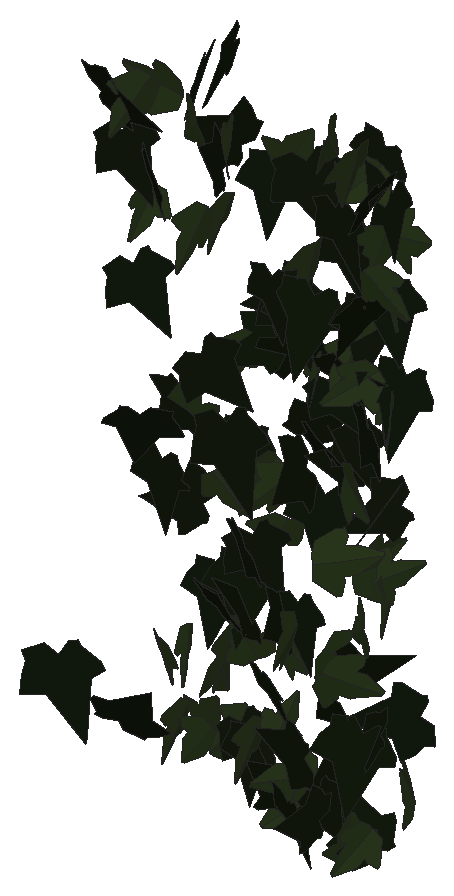
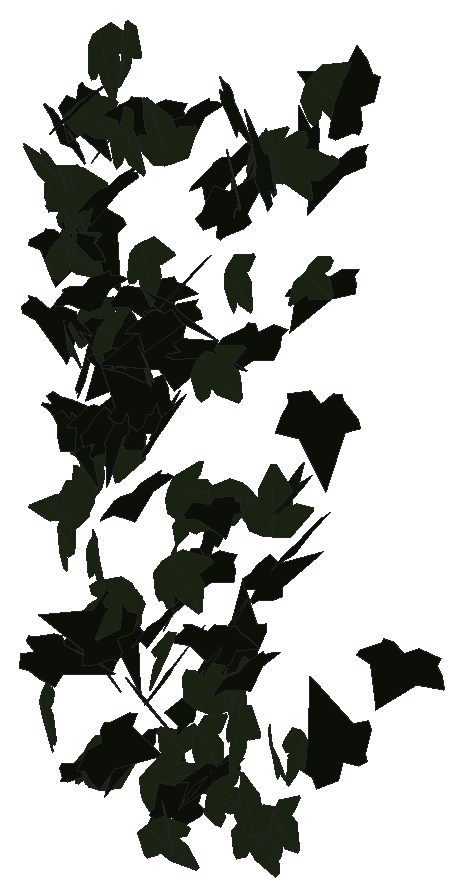
# SketchUp Ruby script. Lengths in inches.
U = 1.inch
M = Sketchup.active_model
def pt(a) = Geom::Point3d.new(a.map { |v| v * U })
def face(e, loops, mat)
  f = e.add_face(loops[0].map { |a| pt(a) })
  loops[1..].each { |l| e.add_face(l.map { |a| pt(a) }).erase! }
  f.material = f.back_material = mat if mat
  f
end
# faces: each face lists its corners as indices into pts; further lists are holes
def faces(e, pts, list, mat = nil) = list.each { |f| face(e, (f[0].is_a?(Array) ? f : [f]).map { |l| l.map { |i| pts[i] } }, mat) }
# xy, xz, yz: faces in a plane at the given z, y or x. An outline is a flat list of corners, or four numbers for a rectangle; further outlines are holes
def ring(l) = l.size == 4 ? [[l[0], l[1]], [l[2], l[1]], [l[2], l[3]], [l[0], l[3]]] : l.each_slice(2).to_a
def flat(e, list, mat, &to3) = list.each { |f| face(e, (f[0].is_a?(Array) ? f : [f]).map { |l| ring(l).map { |u, v| to3.(u, v) } }, mat) }
def xy(e, z, list, mat = nil) = flat(e, list, mat) { |x, y| [x, y, z] }
def xz(e, y, list, mat = nil) = flat(e, list, mat) { |x, z| [x, y, z] }
def yz(e, x, list, mat = nil) = flat(e, list, mat) { |y, z| [x, y, z] }
def lines(e, pts, list) = list.each { |a, b| e.add_line(pt(pts[a]), pt(pts[b])) }
# prism: a flat outline (further loops are holes) pulled along v
def prism(e, loops, v, mat = nil)
  f = face(e, loops, mat); d = Geom::Vector3d.new(v.map { |x| x * U })
  f.pushpull(f.normal.samedirection?(d) ? d.length : -d.length)
end
def box(e, o, s, mat = nil) = prism(e, [[o, [o[0] + s[0], o[1], o[2]], [o[0] + s[0], o[1] + s[1], o[2]], [o[0], o[1] + s[1], o[2]]]], [0, 0, s[2]], mat)
def at(x, y, z, deg = 0) = Geom::Transformation.translation(pt([x, y, z])) * Geom::Transformation.rotation(ORIGIN, Z_AXIS, deg.degrees)
def axes(o, x, y, z) = Geom::Transformation.new([*x, 0, *y, 0, *z, 0, *pt(o).to_a, 1])
def part(name) = M.definitions.add(name)
# library, detail: a bought-in or finely detailed component or shape, given as its bounding box
def library(name, o, s) = part(name).tap { |d| box(d.entities, o, s) }
def detail(e, o, s) = box(e.add_group.entities, o, s)
def put(e, d, t, mat = nil) = e.add_instance(d, t).tap { |i| i.material = mat if mat }
def group(e, t, mat = nil) = e.add_group.tap { |g| g.transformation = t; g.material = mat if mat }.entities
root = M.entities
M.materials.add("efeu1").color = [18, 25, 13]
M.materials.add("efeu2").color = [43, 57, 29]
c1 = part("ivyleaf_9")
p = [[1.54,2.16,1.25],[1.36,2.04,1.19],[-0.21,0.99,0.68],[-0.71,1.11,0.82],[-0.85,0.86,0.67],[-0.8,0.17,0.21],
  [-0.9,-0.01,0.1],[-0.67,-0.16,-0.02],[-0.08,-0.08,-0.05],[-0.03,-0.6,-0.4],[0.65,-0.88,-0.66],[0.83,-0.6,-0.49],
  [1.29,-0.42,-0.43],[1.8125,-0.07,-0.26],[1.21,0.44,0.15]]
faces(c1.entities,p,[[0,1,2,3,4,5,6,7,8,9,10,11,12,13,14]],"efeu1")
c2 = part("ivyleaf_10")
p = [[0,0.5,-0.03],[-0.0625,2.02,-0.43],[-0.19,2.01,-0.46],[-0.54,1.05,-0.29],[-0.52,0.625,-0.18],[-0.83,0.76,-0.28],
  [-1.16,0.64,-0.33],[-1.15,0.33,-0.24],[-0.77,-0.39,0.02],[-0.3,-0.51,0.16],[0.04,-0.48,0.23],[-0.02,2.01,-0.4375],
  [-0.06,2.01,-0.43],[0.04,-0.49,0.23],[0.67,-0.49,0.14],[1.38,0.36,-0.2],[1.375,0.51,-0.24],[0.81,0.65,-0.19],
  [0.62,0.59,-0.15],[0.6,1.09,-0.28],[0.5,1.23,-0.31]]
faces(c2.entities,p,[[0,1,2,3,4,5,6,7,8,9,10],[11,12,0,13,14,15,16,17,18,19,20]],"efeu2")
put(root,c1,axes([563.77,116.41,232.32],[0.19982,-1.30026,-0.40579],[-0.0199,0.4073,-1.3149],[1.36196,0.19672,0.04032]))
put(root,c1,axes([551.59,120.48,215.23],[-0.4996,-0.69607,-0.93578],[0.56579,0.74556,-0.85664],[1.01985,-0.75461,0.01683]))
put(root,c2,axes([557.49,122.375,237.33],[-0.03225,-0.86797,0.78278],[0.26428,-0.76821,-0.84092],[1.13853,0.15373,0.21737]))
put(root,c1,axes([554.65,122.8,237.95],[0.11157,-0.26339,1.12095],[0.35746,-1.06264,-0.28526],[1.09459,0.37387,-0.0211]))
put(root,c1,axes([552.33,122.52,241.55],[0.65037,-0.49363,1.04714],[0.81336,-0.65984,-0.81622],[0.82378,1.04121,-0.02082]))
put(root,c2,axes([553.85,123.06,242.09],[-0.22597,-0.85809,0.7892],[0.00446,-0.80451,-0.87347],[1.16582,-0.16325,0.15632]))
put(root,c1,axes([554.23,122.54,226.77],[0.57412,0.78644,-0.62157],[-0.37365,-0.49678,-0.97368],[-0.93017,0.68496,0.00748]))
put(root,c1,axes([552.55,123.33,211.38],[1.20359,0.26504,-0.0966],[0.08744,0.05198,1.23201],[0.2682,-1.20634,0.03186]))
put(root,c1,axes([563.22,123.0625,210.46],[-0.75467,0.54052,0.38731],[-0.31077,0.23124,-0.92825],[-0.58787,-0.81613,-0.00649]))
put(root,c1,axes([553.4,123.23,233.3],[0.07588,-0.8753,-0.73036],[0.05476,0.73393,-0.87389],[1.13867,0.02304,0.0907]))
put(root,c1,axes([552.61,123.46,239.24],[0.17148,-0.95084,-0.60499],[-0.07155,0.60154,-0.96569],[1.12472,0.18323,0.03081]))
put(root,c2,axes([563.88,124.21,226.11],[0.14329,-0.13167,1.12732],[1.08512,-0.31721,-0.17498],[0.33273,1.09122,0.08517]))
put(root,c1,axes([561.1875,124.55,212.06],[0.33872,-1.06589,-0.12588],[0.0619,-0.11238,1.11814],[-1.07151,-0.34343,0.0248]))
put(root,c2,axes([560.29,124.875,217.49],[0.06922,-0.1292,1.11038],[0.63091,-0.91388,-0.14567],[0.92282,0.63448,0.0163]))
put(root,c1,axes([556.57,123.8,229.89],[0.21395,-0.62477,-0.93815],[-0.06511,0.94645,-0.64515],[1.12526,0.17355,0.14105]))
put(root,c1,axes([559.49,124.8,239.46],[-0.16002,-1.02549,-0.03512],[-0.00159,0.0358,-1.03788],[1.0261,-0.15987,-0.00709]))
put(root,c1,axes([564.03,124.96,213.9],[-0.58748,-1.0267,-0.23131],[0.12138,0.19704,-1.18287],[1.04541,-0.59984,0.00736]))
put(root,c2,axes([563.1,123.8125,222.41],[0.11544,-0.1362,-1.174],[0.94015,0.7254,0.00829],[0.7162,-0.93027,0.17835]))
put(root,c1,axes([557.66,125.22,220.48],[0.05205,-0.53099,0.99543],[0.31094,-0.95115,-0.52363],[1.08451,0.29818,0.10236]))
put(root,c2,axes([563.7,124.87,241.37],[0.07521,-1.21297,0.05991],[0.00537,-0.05969,-1.2153],[1.21444,0.07538,0.00166]))
put(root,c1,axes([562.45,125.29,238.2],[0.50622,-1.09194,-0.01958],[-0.00552,0.01902,-1.20357],[1.0921,0.50624,0.003]))
put(root,c2,axes([562.6,124.54,242.08],[0.21128,-0.76936,-0.68755],[-0.06206,0.69107,-0.79237],[1.02995,0.19947,0.0933]))
put(root,c1,axes([560.21,125.97,224.85],[-0.12803,-0.65853,0.99702],[-0.13719,-0.988,-0.67019],[1.18697,-0.18522,0.03008]))
put(root,c2,axes([563.72,125.6,208.65],[0.33171,0.53207,-0.78016],[-0.40458,-0.66708,-0.62697],[-0.85326,0.52314,-0.006]))
put(root,c2,axes([557.67,125.85,211.58],[0.18836,-0.9537,0.59057],[0.20299,-0.55997,-0.96903],[1.10322,0.26586,0.07747]))
put(root,c1,axes([559.03,126.12,217.18],[-0.12239,-0.40033,0.93488],[-0.01944,-0.94054,-0.4053],[1.01681,-0.06617,0.10479]))
put(root,c1,axes([552.67,125.92,222.57],[0.15073,-1.09674,0.2171],[0.06022,-0.21078,-1.10663],[1.11639,0.15945,0.03039]))
put(root,c1,axes([564.54,125.4,213.9],[-0.87377,0.49225,-0.00129],[0.00171,0.00042,-1.00289],[-0.49225,-0.87377,-0.0012]))
put(root,c2,axes([562.92,125.63,207.91],[-0.40228,-0.88847,-0.15277],[-0.0398,-0.14962,0.97498],[-0.90063,0.40347,0.02515]))
put(root,c2,axes([552.18,125.81,235.1],[0.2298,0.77284,-0.59729],[-0.23902,-0.55045,-0.80419],[-0.94705,0.32645,0.05803]))
put(root,c1,axes([560.77,125.5,239.74],[-0.25873,-0.85282,-0.81291],[0.30819,0.75431,-0.88944],[1.13717,-0.39846,0.0561]))
put(root,c2,axes([555.08,125.16,239.77],[-0.55576,0.28526,0.81128],[-0.76724,0.27184,-0.62117],[-0.38844,-0.94506,0.0662]))
put(root,c1,axes([562.29,125.25,214.91],[0.29107,0.14839,-0.92399],[-0.91838,-0.14072,-0.3119],[-0.17989,0.95848,0.09726]))
put(root,c2,axes([556.18,125.39,223.21],[-0.79403,-0.16262,-0.51737],[0.51351,0.06961,-0.80998],[0.17444,-0.94515,0.02936]))
put(root,c1,axes([559.27,126.08,208.48],[0.50304,-0.86687,0.5011],[0.22328,-0.44955,-1.00183],[0.97607,0.54959,-0.02908]))
put(root,c2,axes([562.47,125.1,216.16],[-0.48111,-0.36705,-0.98062],[0.76698,0.61111,-0.60504],[0.71279,-0.90532,-0.01084]))
put(root,c1,axes([555.4,126.16,216.53],[0.98809,-0.38188,-0.22943],[0.23081,-0.03862,1.05832],[-0.38105,-1.01364,0.04611]))
put(root,c1,axes([561.43,125.46,209.96],[0.30897,-0.65489,-0.66012],[-0.25214,0.61055,-0.72372],[0.89503,0.39808,0.024]))
put(root,c1,axes([563.125,126.47,227.53],[0.5642,-0.45128,-0.97687],[0.88386,-0.43479,0.71134],[-0.61378,-1.04094,0.12639]))
put(root,c1,axes([555.47,126.33,237.32],[-0.22451,0.1807,1.00874],[-0.18831,-1.02236,0.14123],[1.00735,-0.15084,0.25123]))
put(root,c2,axes([556.94,126.34,229.45],[-0.28703,-0.83052,0.66541],[-0.12872,-0.65704,-0.87559],[1.05639,-0.30572,0.07411]))
put(root,c2,axes([555.85,126.36,215.04],[0.33621,-0.87304,0.59235],[0.30026,-0.51681,-0.93213],[1.01139,0.44365,0.07982]))
put(root,c1,axes([565.04,126.18,224.6875],[-0.93567,-0.01956,0.33119],[-0.33126,0.00041,-0.93585],[0.0183,-0.99255,-0.00692]))
put(root,c2,axes([558.25,126.6875,223.21],[-0.09812,-0.34448,1.00567],[-0.02972,-1.00866,-0.34841],[1.06262,-0.06002,0.08312]))
put(root,c1,axes([558.18,126.34,233.02],[0.23801,-0.9804,0.11826],[0.06002,-0.10706,-1.00834],[0.98568,0.24325,0.03284]))
put(root,c2,axes([563.95,125.92,235.2],[-0.7614,0.07192,-0.74112],[0.73273,-0.11617,-0.76406],[-0.13244,-1.05617,0.03357]))
put(root,c1,axes([563.37,126.09,233.74],[-0.13607,0.85879,-0.68034],[0.12597,-0.66876,-0.86936],[-1.08835,-0.18477,-0.01556]))
put(root,c1,axes([563.86,126.27,239.27],[-0.45295,0.68125,-0.58517],[0.28933,-0.50975,-0.81739],[-0.85018,-0.53642,0.03359]))
put(root,c2,axes([552.88,126.14,240.24],[-0.29806,0.07463,-1.10758],[-1.09936,0.13924,0.30523],[0.154,1.1385,0.03528]))
put(root,c1,axes([556.83,126.65,210.47],[0.04703,-0.9871,0.13749],[0.00014,-0.13763,-0.9882],[0.99663,0.0466,-0.00635]))
put(root,c2,axes([563.75,125.38,221.38],[0.04397,0.12404,0.98906],[-0.21044,0.96886,-0.11215],[-0.97434,-0.20366,0.06885]))
put(root,c2,axes([563.48,125.78,218.42],[-0.40323,0.32257,0.85143],[-0.80553,0.30764,-0.49805],[-0.42438,-0.89044,0.13637]))
put(root,c1,axes([563.57,126.24,208.01],[-0.78821,-0.6818,0.16491],[0.1283,0.10375,1.04216],[-0.68963,0.79857,0.00541]))
put(root,c1,axes([557.96,126.77,229.95],[-0.79645,-0.32253,0.45284],[-0.41806,-0.17408,-0.85927],[0.36649,-0.89949,0.00392]))
put(root,c2,axes([559.16,127.1,209.35],[0.00767,0.20492,1.16685],[-0.19926,-1.15002,0.20328],[1.16783,-0.19757,0.02702]))
put(root,c2,axes([562.93,126.72,229.78],[0.44622,0.3457,-0.90075],[-0.76087,-0.48413,-0.56273],[-0.59324,0.88095,0.04422]))
put(root,c1,axes([553.83,127.03,220.54],[-0.27838,-0.10978,0.97763],[-0.75822,-0.62342,-0.28591],[0.62682,-0.80287,0.08833]))
put(root,c1,axes([560.01,126.8,225.55],[0.23101,-0.38457,0.85517],[0.56804,-0.64333,-0.44275],[0.74601,0.60894,0.07232]))
put(root,c2,axes([561.64,125.93,216.74],[-0.20892,-0.62362,-0.72993],[0.33646,0.65207,-0.65341],[0.89916,-0.3889,0.0749]))
put(root,c1,axes([564.17,126.3,224.25],[-0.53143,0.81805,-0.2085],[0.12309,-0.16865,-0.97545],[-0.83518,-0.54539,-0.0111]))
put(root,c1,axes([557.44,126.73,213.6],[0.57205,-0.69663,0.32705],[0.19694,-0.26141,-0.90131],[0.74395,0.60487,-0.01287]))
put(root,c2,axes([559.04,126.5,238.86],[-0.92014,-0.36627,0.49589],[0.46119,0.18226,0.99036],[-0.40911,1.02925,0.0011]))
put(root,c1,axes([552.64,127.4,224.7],[-0.38175,-0.62867,0.8567],[0.15762,-0.93373,-0.61496],[1.05086,-0.08833,0.40345]))
put(root,c1,axes([557.17,126.38,220.35],[-0.14022,-0.67733,-0.78077],[0.1312,0.76989,-0.69145],[1.02527,-0.19115,-0.0183]))
put(root,c1,axes([558.28,127,208.39],[0.21313,0.20583,0.91622],[-0.7223,-0.56446,0.29483],[0.60009,-0.75251,0.02946]))
put(root,c1,axes([559.74,127.0625,232.31],[-0.63954,-0.98527,-0.24235],[0.13303,0.20257,-1.17464],[1.00588,-0.65323,0.00126]))
put(root,c2,axes([552.29,126.41,213.5],[-0.78997,0.50222,0.00553],[-0.00483,0.0027,-0.9361],[-0.50223,-0.78999,0.00031]))
put(root,c1,axes([556.47,127.08,216.09],[0.36636,-0.96597,0.06594],[0.00945,0.07406,1.03252],[-0.96818,-0.3648,0.03503]))
put(root,c1,axes([561.81,126.86,236.25],[0.17964,-1.05627,-0.2565],[-0.02264,0.25628,-1.07125],[1.08673,0.17994,0.02008]))
put(root,c2,axes([552.66,127.19,210.07],[0.20709,-0.85,0.63633],[0.24214,-0.59343,-0.8715],[1.03382,0.30926,0.07665]))
put(root,c2,axes([561.6,126.32,238.84],[-0.38622,0.06365,1.14036],[-1.10847,0.26922,-0.39045],[-0.27525,-1.1735,-0.02772]))
put(root,c2,axes([562.96,126.97,239.42],[0.60172,0.38608,-0.75551],[-0.67657,-0.34054,-0.71287],[-0.51195,0.90382,0.05413]))
put(root,c2,axes([556,126.1,238.29],[0.14046,-0.01361,1.16168],[-0.99376,0.60472,0.12725],[-0.60178,-1.00178,0.06103]))
put(root,c2,axes([556.59,127.07,214.42],[-0.74717,-0.55654,-0.45091],[-0.36336,-0.26701,0.93167],[-0.61728,0.83084,-0.00263]))
put(root,c2,axes([563.66,127.14,228.77],[0.63125,-0.36967,0.66999],[0.5602,-0.36841,-0.73108],[0.52127,0.84359,-0.02567]))
put(root,c2,axes([559.95,127.03,229.36],[0.71016,-0.58761,0.30462],[0.23306,-0.19618,-0.92174],[0.61949,0.74742,-0.00244]))
put(root,c1,axes([556.37,126.7,211.05],[0.19254,-0.78435,-0.58696],[0.08268,0.60906,-0.78677],[0.97616,0.10312,0.18241]))
put(root,c1,axes([560.14,127.35,222.83],[-0.07075,-1.18144,-0.0314],[0.00218,0.03133,-1.18355],[1.18185,-0.07078,0.0003]))
put(root,c1,axes([563.87,127.25,238.57],[-0.43883,-0.31892,-0.83636],[0.88099,0.01089,-0.46639],[0.15834,-0.94443,0.27705]))
put(root,c1,axes([561.37,127.7,210.87],[-0.02952,-0.06564,-1.18238],[0.37849,-1.12123,0.0528],[-1.12208,-0.37647,0.04891]))
put(root,c1,axes([560.98,126.875,229.15],[0.38396,-0.25382,0.87054],[0.82926,-0.28418,-0.44861],[0.36686,0.90802,0.10294]))
put(root,c1,axes([560.07,126.66,226.36],[-0.21244,-0.2107,0.91996],[0.9425,0.00185,0.21807],[-0.04925,0.94417,0.20487]))
put(root,c2,axes([561.375,127.57,230],[-0.20151,-0.6161,0.84039],[0.36128,-0.84418,-0.53224],[0.9774,0.18501,0.37]))
put(root,c1,axes([558.85,127.24,217.32],[0.21717,-1.00721,-0.05802],[-0.00831,0.05756,-1.03035],[1.00885,0.21729,0.004]))
put(root,c2,axes([559.09,126.39,215.77],[-0.28508,0.75096,0.54197],[-0.19494,0.5057,-0.80325],[-0.90536,-0.34535,0.0023]))
put(root,c1,axes([555.46,127.15,242.88],[-0.80084,0.39954,-0.55784],[0.50684,-0.2335,-0.89485],[-0.46253,-0.94764,-0.0147]))
put(root,c2,axes([555.16,126.61,213.71],[0.11681,-1.01962,-0.54688],[0.03993,0.55289,-1.02229],[1.15634,0.08391,0.09055]))
put(root,c1,axes([561.76,127.67,224.83],[-0.18208,-0.06798,1.00578],[-0.6817,-0.74464,-0.17374],[0.74264,-0.70019,0.08711]))
put(root,c2,axes([563.51,127.625,219.92],[0.31043,-0.7438,0.84573],[0.56758,-0.65442,-0.78387],[0.97281,0.61916,0.18747]))
put(root,c2,axes([554.78,127.49,234.87],[0.24057,-0.90348,0.49968],[0.17335,-0.47043,-0.93406],[1.0178,0.29368,0.04098]))
put(root,c2,axes([563.76,126.36,220.66],[0.08341,0.08855,-1.05482],[0.69422,0.79418,0.12157],[0.79909,-0.6992,0.00449]))
put(root,c1,axes([561.75,126.6,215.24],[0.29957,0.02723,1.04417],[1.02175,0.21799,-0.29882],[-0.21696,1.0642,0.03449]))
put(root,c1,axes([558.43,126.53,230.19],[0.11075,0.16813,-1.16674],[0.60456,0.99792,0.20119],[1.01196,-0.61458,0.0075]))
put(root,c2,axes([555.4375,127.76,210.48],[-0.09444,-0.43705,0.83311],[0.01269,-0.83781,-0.43807],[0.9407,-0.03257,0.08955]))
put(root,c2,axes([563.34,127.71,233.23],[-0.53256,-0.50496,0.77421],[-0.22803,-0.79413,-0.67481],[0.89576,-0.50238,0.28851]))
put(root,c1,axes([564.32,127.47,229.9],[-0.94663,-0.4547,-0.58605],[0.52281,0.26504,-1.05012],[0.52619,-1.08135,-0.01096]))
put(root,c2,axes([552.87,127.35,224.08],[-0.91698,-0.72204,-0.07403],[-0.05214,-0.05344,1.1671],[-0.72395,0.91841,0.00971]))
put(root,c2,axes([558.24,126.58,211.27],[0.27407,0.65025,-0.65052],[0.25464,0.59861,0.70564],[0.88383,-0.3741,-0.00158]))
put(root,c1,axes([558.88,127.26,232.06],[-0.81432,0.30247,0.44741],[-0.45831,0.04118,-0.862],[-0.28568,-0.92822,0.10755]))
put(root,c2,axes([552.7,127.51,213.59],[0.70616,-0.52767,0.49458],[0.41417,-0.27161,-0.88113],[0.59288,0.81822,0.02646]))
put(root,c2,axes([557.02,127.71,223.1],[0.16281,0.53463,-0.77905],[-0.36018,-0.69572,-0.55271],[-0.87351,0.38652,0.0827]))
put(root,c1,axes([554.2,127.8,216.78],[-0.1482,-1.05499,0.11095],[-0.01403,-0.11006,-1.06535],[1.06072,-0.14886,0.00141]))
put(root,c1,axes([555.99,127.63,217.9],[-0.76612,-0.78868,-0.4173],[0.30949,0.28099,-1.09925],[0.83688,-0.8259,0.0245]))
put(root,c1,axes([553.22,127.22,239.5625],[-0.17219,0.88675,0.7018],[0.01738,-0.70773,0.89851],[1.13073,0.14591,0.09306]))
put(root,c1,axes([564.81,127.6875,213.92],[-0.28167,-0.37531,-1.00841],[-0.64128,-0.77847,0.46886],[-0.864,0.70015,-0.01924]))
put(root,c1,axes([560.8125,127.11,228.6],[-0.15157,-0.48267,-0.84014],[0.40413,0.74136,-0.49883],[0.88062,-0.4233,0.08432]))
put(root,c2,axes([558.6,127.26,208.71],[0.56691,-0.79841,-0.18709],[-0.0829,0.17048,-0.97873],[0.81583,0.57213,0.03055]))
put(root,c2,axes([563.3125,126.56,221.2],[0.13167,-0.22042,0.96227],[-0.10525,0.96213,0.23479],[-0.98157,-0.13273,0.1039]))
put(root,c2,axes([553.87,127.46,209.37],[-0.75017,-0.2958,0.61772],[-0.55127,-0.28289,-0.80493],[0.40643,-0.92968,0.04838]))
put(root,c1,axes([558.33,127.53,231.87],[-0.0767,-1.02867,-0.49097],[0.09279,0.48481,-1.03026],[1.13605,-0.10905,0.051]))
put(root,c2,axes([565.1875,126.7,210.72],[0.08464,-0.13184,-1.20356],[-0.68951,0.98649,-0.15655],[0.99524,0.69466,-0.00611]))
put(root,c1,axes([562.71,128.12,240.01],[-0.11356,-0.95344,0.41896],[0.05541,-0.42638,-0.9553],[1.03995,-0.08139,0.09664]))
put(root,c2,axes([563.28,127.57,234.05],[-0.66233,0.54916,-0.48793],[0.30033,-0.39713,-0.85465],[-0.67041,-0.72045,0.09919]))
put(root,c2,axes([553.77,127.53,209.79],[-0.91607,0.04496,0.43505],[0.4349,-0.01342,0.91715],[0.04638,1.01404,-0.00715]))
put(root,c2,axes([559.38,127.55,234.27],[-0.1129,-1.04631,0.02761],[0.00032,-0.0278,-1.05238],[1.04668,-0.11286,0.0033]))
put(root,c2,axes([563.15,127.625,236.29],[-0.62951,-0.76609,0.26512],[-0.15428,-0.21632,-0.9914],[0.79585,-0.6479,0.01752]))
put(root,c1,axes([555.03,128.09,237.62],[0.0017,0.11962,1.08392],[-0.83561,-0.69631,0.07815],[0.70068,-0.83069,0.09057]))
put(root,c1,axes([561.1875,127.02,225.77],[0.54378,0.13295,-0.79417],[-0.80267,0.16577,-0.52185],[0.06409,0.94812,0.20261]))
put(root,c2,axes([557.58,127.79,220.4],[-0.53464,-0.74223,0.50533],[-0.30667,-0.40182,-0.91466],[0.84393,-0.61623,-0.01224]))
put(root,c1,axes([561.74,127.54,226.31],[0.12192,-0.85642,-0.46133],[-0.02656,0.46184,-0.86438],[0.97241,0.11999,0.03424]))
put(root,c1,axes([563.45,127.64,233.62],[-0.515,-0.678,-0.63615],[0.36147,0.52399,-0.85109],[0.85657,-0.62876,-0.02332]))
put(root,c1,axes([562.14,128.01,232.05],[-0.35442,-0.99544,-0.08466],[0.03108,0.0788,-1.05665],[0.99855,-0.35577,0.00284]))
put(root,c1,axes([555.65,127.91,224.08],[-0.54251,-0.74393,-0.21149],[0.12479,0.17075,-0.92073],[0.76327,-0.55668,0.00021]))
put(root,c2,axes([563.78,127.82,236.4],[0.18661,-0.23896,-1.05542],[0.9361,-0.50166,0.27909],[-0.54289,-0.94714,0.11845]))
put(root,c2,axes([558.59,127.7,207.69],[0.72558,0.09793,-0.76954],[-0.76432,-0.08995,-0.7321],[-0.13267,1.05384,0.00903]))
